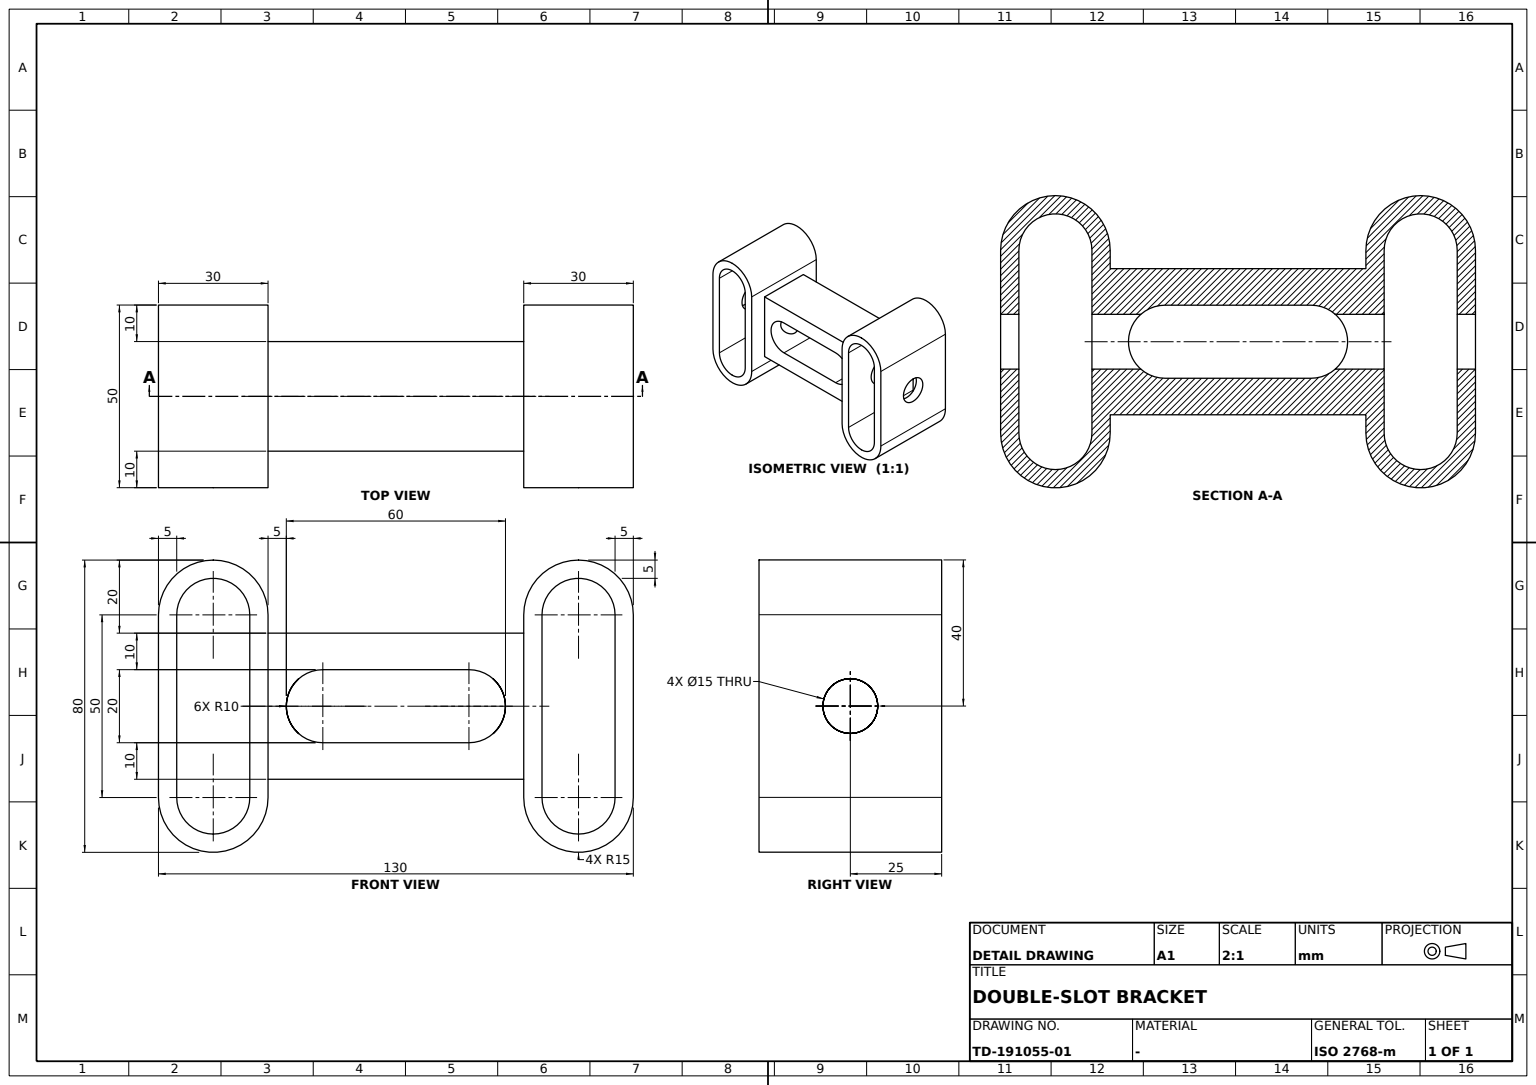
ISO-10303-21;
HEADER;
FILE_DESCRIPTION((''),'2;1');
FILE_NAME('','',(''),(''),'','','');
FILE_SCHEMA(('AUTOMOTIVE_DESIGN'));
ENDSEC;
DATA;
#1=APPLICATION_CONTEXT('');
#2=PRODUCT_CONTEXT('',#1,'mechanical');
#3=PRODUCT('','','',(#2));
#4=PRODUCT_DEFINITION_FORMATION('','',#3);
#5=PRODUCT_DEFINITION_CONTEXT('',#1,'design');
#6=PRODUCT_DEFINITION('','',#4,#5);
#7=PRODUCT_DEFINITION_SHAPE('','',#6);
#8=(LENGTH_UNIT()NAMED_UNIT(*)SI_UNIT(.MILLI.,.METRE.));
#9=(NAMED_UNIT(*)PLANE_ANGLE_UNIT()SI_UNIT($,.RADIAN.));
#10=(NAMED_UNIT(*)SI_UNIT($,.STERADIAN.)SOLID_ANGLE_UNIT());
#11=UNCERTAINTY_MEASURE_WITH_UNIT(LENGTH_MEASURE(0.005),#8,'distance_accuracy_value','');
#12=(GEOMETRIC_REPRESENTATION_CONTEXT(3)GLOBAL_UNCERTAINTY_ASSIGNED_CONTEXT((#11))GLOBAL_UNIT_ASSIGNED_CONTEXT((#8,#9,#10))REPRESENTATION_CONTEXT('',''));
#13=CARTESIAN_POINT('',(60.,-25.,25.));
#14=VERTEX_POINT('',#13);
#15=CARTESIAN_POINT('',(40.,-25.,25.));
#16=VERTEX_POINT('',#15);
#17=CARTESIAN_POINT('',(50.,-25.,25.));
#18=DIRECTION('',(0.,-1.,0.));
#19=DIRECTION('',(1.,0.,0.));
#20=AXIS2_PLACEMENT_3D('',#17,#18,#19);
#21=CIRCLE('',#20,10.);
#22=EDGE_CURVE('',#14,#16,#21,.T.);
#23=ORIENTED_EDGE('',*,*,#22,.F.);
#24=CARTESIAN_POINT('',(60.,-25.,-25.));
#25=VERTEX_POINT('',#24);
#26=DIRECTION('',(0.,0.,1.));
#27=VECTOR('',#26,1000.);
#28=LINE('',#24,#27);
#29=EDGE_CURVE('',#25,#14,#28,.T.);
#30=ORIENTED_EDGE('',*,*,#29,.F.);
#31=CARTESIAN_POINT('',(50.,-25.,-35.));
#32=VERTEX_POINT('',#31);
#33=CARTESIAN_POINT('',(50.,-25.,-25.));
#34=AXIS2_PLACEMENT_3D('',#33,#18,#19);
#35=CIRCLE('',#34,10.);
#36=EDGE_CURVE('',#32,#25,#35,.T.);
#37=ORIENTED_EDGE('',*,*,#36,.F.);
#38=CARTESIAN_POINT('',(40.,-25.,-25.));
#39=VERTEX_POINT('',#38);
#40=EDGE_CURVE('',#39,#32,#35,.T.);
#41=ORIENTED_EDGE('',*,*,#40,.F.);
#42=DIRECTION('',(0.,0.,-1.));
#43=VECTOR('',#42,1000.);
#44=LINE('',#15,#43);
#45=EDGE_CURVE('',#16,#39,#44,.T.);
#46=ORIENTED_EDGE('',*,*,#45,.F.);
#47=EDGE_LOOP('',(#23,#30,#37,#41,#46));
#48=FACE_BOUND('',#47,.T.);
#49=CARTESIAN_POINT('',(50.,-25.,40.));
#50=VERTEX_POINT('',#49);
#51=CARTESIAN_POINT('',(35.,-25.,25.));
#52=VERTEX_POINT('',#51);
#53=CIRCLE('',#20,15.);
#54=EDGE_CURVE('',#50,#52,#53,.T.);
#55=ORIENTED_EDGE('',*,*,#54,.T.);
#56=CARTESIAN_POINT('',(35.,-25.,-25.));
#57=VERTEX_POINT('',#56);
#58=LINE('',#51,#43);
#59=EDGE_CURVE('',#52,#57,#58,.T.);
#60=ORIENTED_EDGE('',*,*,#59,.T.);
#61=CARTESIAN_POINT('',(65.,-25.,-25.));
#62=VERTEX_POINT('',#61);
#63=CIRCLE('',#34,15.);
#64=EDGE_CURVE('',#57,#62,#63,.T.);
#65=ORIENTED_EDGE('',*,*,#64,.T.);
#66=CARTESIAN_POINT('',(65.,-25.,25.));
#67=VERTEX_POINT('',#66);
#68=LINE('',#61,#27);
#69=EDGE_CURVE('',#62,#67,#68,.T.);
#70=ORIENTED_EDGE('',*,*,#69,.T.);
#71=EDGE_CURVE('',#67,#50,#53,.T.);
#72=ORIENTED_EDGE('',*,*,#71,.T.);
#73=EDGE_LOOP('',(#55,#60,#65,#70,#72));
#74=FACE_BOUND('',#73,.T.);
#75=AXIS2_PLACEMENT_3D('',#33,#18,#42);
#76=PLANE('',#75);
#77=ADVANCED_FACE('',(#48,#74),#76,.T.);
#78=CARTESIAN_POINT('',(-60.,-25.,-25.));
#79=VERTEX_POINT('',#78);
#80=CARTESIAN_POINT('',(-60.,25.,-25.));
#81=VERTEX_POINT('',#80);
#82=DIRECTION('',(0.,1.,0.));
#83=VECTOR('',#82,1000.);
#84=LINE('',#80,#83);
#85=EDGE_CURVE('',#79,#81,#84,.T.);
#86=ORIENTED_EDGE('',*,*,#85,.T.);
#87=CARTESIAN_POINT('',(-60.,25.,25.));
#88=VERTEX_POINT('',#87);
#89=LINE('',#87,#43);
#90=EDGE_CURVE('',#88,#81,#89,.T.);
#91=ORIENTED_EDGE('',*,*,#90,.F.);
#92=CARTESIAN_POINT('',(-60.,-25.,25.));
#93=VERTEX_POINT('',#92);
#94=LINE('',#87,#83);
#95=EDGE_CURVE('',#93,#88,#94,.T.);
#96=ORIENTED_EDGE('',*,*,#95,.F.);
#97=LINE('',#92,#43);
#98=EDGE_CURVE('',#93,#79,#97,.T.);
#99=ORIENTED_EDGE('',*,*,#98,.T.);
#100=EDGE_LOOP('',(#86,#91,#96,#99));
#101=FACE_BOUND('',#100,.T.);
#102=CARTESIAN_POINT('',(-60.,0.,7.5));
#103=VERTEX_POINT('',#102);
#104=CARTESIAN_POINT('',(-60.,0.,-7.5));
#105=VERTEX_POINT('',#104);
#106=CARTESIAN_POINT('',(-60.,0.,0.));
#107=DIRECTION('',(-1.,0.,0.));
#108=AXIS2_PLACEMENT_3D('',#106,#107,#26);
#109=CIRCLE('',#108,7.5);
#110=EDGE_CURVE('',#103,#105,#109,.T.);
#111=ORIENTED_EDGE('',*,*,#110,.T.);
#112=EDGE_CURVE('',#105,#103,#109,.T.);
#113=ORIENTED_EDGE('',*,*,#112,.T.);
#114=EDGE_LOOP('',(#111,#113));
#115=FACE_BOUND('',#114,.T.);
#116=AXIS2_PLACEMENT_3D('',#87,#107,#26);
#117=PLANE('',#116);
#118=ADVANCED_FACE('',(#101,#115),#117,.F.);
#119=ORIENTED_EDGE('',*,*,#64,.F.);
#120=CARTESIAN_POINT('',(35.,25.,-25.));
#121=VERTEX_POINT('',#120);
#122=LINE('',#56,#83);
#123=EDGE_CURVE('',#57,#121,#122,.T.);
#124=ORIENTED_EDGE('',*,*,#123,.T.);
#125=CARTESIAN_POINT('',(65.,25.,-25.));
#126=VERTEX_POINT('',#125);
#127=CARTESIAN_POINT('',(50.,25.,-25.));
#128=AXIS2_PLACEMENT_3D('',#127,#18,#19);
#129=CIRCLE('',#128,15.);
#130=EDGE_CURVE('',#121,#126,#129,.T.);
#131=ORIENTED_EDGE('',*,*,#130,.T.);
#132=LINE('',#61,#83);
#133=EDGE_CURVE('',#62,#126,#132,.T.);
#134=ORIENTED_EDGE('',*,*,#133,.F.);
#135=EDGE_LOOP('',(#119,#124,#131,#134));
#136=FACE_BOUND('',#135,.T.);
#137=AXIS2_PLACEMENT_3D('',#33,#82,#26);
#138=CYLINDRICAL_SURFACE('',#137,15.);
#139=ADVANCED_FACE('',(#136),#138,.T.);
#140=CARTESIAN_POINT('',(-65.,0.,-7.5));
#141=VERTEX_POINT('',#140);
#142=CARTESIAN_POINT('',(-54935.,0.,-7.5));
#143=VECTOR('',#19,1000.);
#144=LINE('',#142,#143);
#145=EDGE_CURVE('',#141,#105,#144,.T.);
#146=ORIENTED_EDGE('',*,*,#145,.T.);
#147=ORIENTED_EDGE('',*,*,#110,.F.);
#148=CARTESIAN_POINT('',(-65.,0.,7.5));
#149=VERTEX_POINT('',#148);
#150=CARTESIAN_POINT('',(-54935.,0.,7.5));
#151=LINE('',#150,#143);
#152=EDGE_CURVE('',#103,#149,#151,.F.);
#153=ORIENTED_EDGE('',*,*,#152,.T.);
#154=CARTESIAN_POINT('',(-65.,0.,0.));
#155=AXIS2_PLACEMENT_3D('',#154,#19,#42);
#156=CIRCLE('',#155,7.5);
#157=EDGE_CURVE('',#141,#149,#156,.T.);
#158=ORIENTED_EDGE('',*,*,#157,.F.);
#159=EDGE_LOOP('',(#146,#147,#153,#158));
#160=FACE_BOUND('',#159,.T.);
#161=CARTESIAN_POINT('',(-54935.,0.,0.));
#162=AXIS2_PLACEMENT_3D('',#161,#19,#42);
#163=CYLINDRICAL_SURFACE('',#162,7.5);
#164=ADVANCED_FACE('',(#160),#163,.F.);
#165=CARTESIAN_POINT('',(-35.,-25.,-25.));
#166=VERTEX_POINT('',#165);
#167=CARTESIAN_POINT('',(-35.,25.,-25.));
#168=VERTEX_POINT('',#167);
#169=LINE('',#165,#83);
#170=EDGE_CURVE('',#166,#168,#169,.T.);
#171=ORIENTED_EDGE('',*,*,#170,.T.);
#172=CARTESIAN_POINT('',(-35.,25.,25.));
#173=VERTEX_POINT('',#172);
#174=LINE('',#167,#27);
#175=EDGE_CURVE('',#168,#173,#174,.T.);
#176=ORIENTED_EDGE('',*,*,#175,.T.);
#177=CARTESIAN_POINT('',(-35.,-25.,25.));
#178=VERTEX_POINT('',#177);
#179=LINE('',#177,#83);
#180=EDGE_CURVE('',#178,#173,#179,.T.);
#181=ORIENTED_EDGE('',*,*,#180,.F.);
#182=LINE('',#165,#27);
#183=EDGE_CURVE('',#166,#178,#182,.T.);
#184=ORIENTED_EDGE('',*,*,#183,.F.);
#185=EDGE_LOOP('',(#171,#176,#181,#184));
#186=FACE_BOUND('',#185,.T.);
#187=CARTESIAN_POINT('',(-35.,-15.,20.));
#188=VERTEX_POINT('',#187);
#189=CARTESIAN_POINT('',(-35.,-15.,-20.));
#190=VERTEX_POINT('',#189);
#191=LINE('',#187,#43);
#192=EDGE_CURVE('',#188,#190,#191,.T.);
#193=ORIENTED_EDGE('',*,*,#192,.F.);
#194=CARTESIAN_POINT('',(-35.,15.,20.));
#195=VERTEX_POINT('',#194);
#196=LINE('',#187,#83);
#197=EDGE_CURVE('',#188,#195,#196,.T.);
#198=ORIENTED_EDGE('',*,*,#197,.T.);
#199=CARTESIAN_POINT('',(-35.,15.,-20.));
#200=VERTEX_POINT('',#199);
#201=LINE('',#194,#43);
#202=EDGE_CURVE('',#195,#200,#201,.T.);
#203=ORIENTED_EDGE('',*,*,#202,.T.);
#204=LINE('',#189,#83);
#205=EDGE_CURVE('',#190,#200,#204,.T.);
#206=ORIENTED_EDGE('',*,*,#205,.F.);
#207=EDGE_LOOP('',(#193,#198,#203,#206));
#208=FACE_BOUND('',#207,.T.);
#209=AXIS2_PLACEMENT_3D('',#165,#107,#26);
#210=PLANE('',#209);
#211=ADVANCED_FACE('',(#186,#208),#210,.F.);
#212=CARTESIAN_POINT('',(60.,0.,-7.5));
#213=VERTEX_POINT('',#212);
#214=CARTESIAN_POINT('',(60.,0.,7.5));
#215=VERTEX_POINT('',#214);
#216=CARTESIAN_POINT('',(60.,0.,0.));
#217=AXIS2_PLACEMENT_3D('',#216,#19,#42);
#218=CIRCLE('',#217,7.5);
#219=EDGE_CURVE('',#213,#215,#218,.T.);
#220=ORIENTED_EDGE('',*,*,#219,.T.);
#221=EDGE_CURVE('',#215,#213,#218,.T.);
#222=ORIENTED_EDGE('',*,*,#221,.T.);
#223=EDGE_LOOP('',(#220,#222));
#224=FACE_BOUND('',#223,.T.);
#225=ORIENTED_EDGE('',*,*,#29,.T.);
#226=CARTESIAN_POINT('',(60.,25.,25.));
#227=VERTEX_POINT('',#226);
#228=LINE('',#226,#83);
#229=EDGE_CURVE('',#14,#227,#228,.T.);
#230=ORIENTED_EDGE('',*,*,#229,.T.);
#231=CARTESIAN_POINT('',(60.,25.,-25.));
#232=VERTEX_POINT('',#231);
#233=LINE('',#231,#27);
#234=EDGE_CURVE('',#232,#227,#233,.T.);
#235=ORIENTED_EDGE('',*,*,#234,.F.);
#236=LINE('',#231,#83);
#237=EDGE_CURVE('',#25,#232,#236,.T.);
#238=ORIENTED_EDGE('',*,*,#237,.F.);
#239=EDGE_LOOP('',(#225,#230,#235,#238));
#240=FACE_BOUND('',#239,.T.);
#241=AXIS2_PLACEMENT_3D('',#231,#19,#42);
#242=PLANE('',#241);
#243=ADVANCED_FACE('',(#224,#240),#242,.F.);
#244=CARTESIAN_POINT('',(65.,0.,7.5));
#245=VERTEX_POINT('',#244);
#246=CARTESIAN_POINT('',(65.,0.,-7.5));
#247=VERTEX_POINT('',#246);
#248=CARTESIAN_POINT('',(65.,0.,0.));
#249=AXIS2_PLACEMENT_3D('',#248,#19,#82);
#250=CIRCLE('',#249,7.5);
#251=EDGE_CURVE('',#245,#247,#250,.T.);
#252=ORIENTED_EDGE('',*,*,#251,.F.);
#253=EDGE_CURVE('',#247,#245,#250,.T.);
#254=ORIENTED_EDGE('',*,*,#253,.F.);
#255=EDGE_LOOP('',(#252,#254));
#256=FACE_BOUND('',#255,.T.);
#257=ORIENTED_EDGE('',*,*,#69,.F.);
#258=ORIENTED_EDGE('',*,*,#133,.T.);
#259=CARTESIAN_POINT('',(65.,25.,25.));
#260=VERTEX_POINT('',#259);
#261=LINE('',#125,#27);
#262=EDGE_CURVE('',#126,#260,#261,.T.);
#263=ORIENTED_EDGE('',*,*,#262,.T.);
#264=LINE('',#66,#83);
#265=EDGE_CURVE('',#67,#260,#264,.T.);
#266=ORIENTED_EDGE('',*,*,#265,.F.);
#267=EDGE_LOOP('',(#257,#258,#263,#266));
#268=FACE_BOUND('',#267,.T.);
#269=AXIS2_PLACEMENT_3D('',#61,#107,#26);
#270=PLANE('',#269);
#271=ADVANCED_FACE('',(#256,#268),#270,.F.);
#272=CARTESIAN_POINT('',(50.,25.,40.));
#273=VERTEX_POINT('',#272);
#274=LINE('',#49,#83);
#275=EDGE_CURVE('',#50,#273,#274,.T.);
#276=ORIENTED_EDGE('',*,*,#275,.F.);
#277=ORIENTED_EDGE('',*,*,#71,.F.);
#278=ORIENTED_EDGE('',*,*,#265,.T.);
#279=CARTESIAN_POINT('',(50.,25.,25.));
#280=AXIS2_PLACEMENT_3D('',#279,#18,#19);
#281=CIRCLE('',#280,15.);
#282=EDGE_CURVE('',#260,#273,#281,.T.);
#283=ORIENTED_EDGE('',*,*,#282,.T.);
#284=EDGE_LOOP('',(#276,#277,#278,#283));
#285=FACE_BOUND('',#284,.T.);
#286=AXIS2_PLACEMENT_3D('',#17,#82,#26);
#287=CYLINDRICAL_SURFACE('',#286,15.);
#288=ADVANCED_FACE('',(#285),#287,.T.);
#289=CARTESIAN_POINT('',(-50.,25.,40.));
#290=VERTEX_POINT('',#289);
#291=CARTESIAN_POINT('',(-65.,25.,25.));
#292=VERTEX_POINT('',#291);
#293=CARTESIAN_POINT('',(-50.,25.,25.));
#294=AXIS2_PLACEMENT_3D('',#293,#18,#19);
#295=CIRCLE('',#294,15.);
#296=EDGE_CURVE('',#290,#292,#295,.T.);
#297=ORIENTED_EDGE('',*,*,#296,.T.);
#298=CARTESIAN_POINT('',(-65.,-25.,25.));
#299=VERTEX_POINT('',#298);
#300=LINE('',#298,#83);
#301=EDGE_CURVE('',#299,#292,#300,.T.);
#302=ORIENTED_EDGE('',*,*,#301,.F.);
#303=CARTESIAN_POINT('',(-50.,-25.,40.));
#304=VERTEX_POINT('',#303);
#305=CARTESIAN_POINT('',(-50.,-25.,25.));
#306=AXIS2_PLACEMENT_3D('',#305,#18,#19);
#307=CIRCLE('',#306,15.);
#308=EDGE_CURVE('',#304,#299,#307,.T.);
#309=ORIENTED_EDGE('',*,*,#308,.F.);
#310=LINE('',#303,#83);
#311=EDGE_CURVE('',#304,#290,#310,.T.);
#312=ORIENTED_EDGE('',*,*,#311,.T.);
#313=EDGE_LOOP('',(#297,#302,#309,#312));
#314=FACE_BOUND('',#313,.T.);
#315=AXIS2_PLACEMENT_3D('',#305,#82,#26);
#316=CYLINDRICAL_SURFACE('',#315,15.);
#317=ADVANCED_FACE('',(#314),#316,.T.);
#318=CARTESIAN_POINT('',(20.,15.,10.));
#319=VERTEX_POINT('',#318);
#320=CARTESIAN_POINT('',(-20.,15.,10.));
#321=VERTEX_POINT('',#320);
#322=VECTOR('',#107,1000.);
#323=LINE('',#318,#322);
#324=EDGE_CURVE('',#319,#321,#323,.T.);
#325=ORIENTED_EDGE('',*,*,#324,.F.);
#326=CARTESIAN_POINT('',(20.,-15.,10.));
#327=VERTEX_POINT('',#326);
#328=LINE('',#318,#83);
#329=EDGE_CURVE('',#327,#319,#328,.T.);
#330=ORIENTED_EDGE('',*,*,#329,.F.);
#331=CARTESIAN_POINT('',(-20.,-15.,10.));
#332=VERTEX_POINT('',#331);
#333=LINE('',#326,#322);
#334=EDGE_CURVE('',#327,#332,#333,.T.);
#335=ORIENTED_EDGE('',*,*,#334,.T.);
#336=LINE('',#320,#83);
#337=EDGE_CURVE('',#332,#321,#336,.T.);
#338=ORIENTED_EDGE('',*,*,#337,.T.);
#339=EDGE_LOOP('',(#325,#330,#335,#338));
#340=FACE_BOUND('',#339,.T.);
#341=AXIS2_PLACEMENT_3D('',#318,#26,#19);
#342=PLANE('',#341);
#343=ADVANCED_FACE('',(#340),#342,.F.);
#344=CARTESIAN_POINT('',(35.,25.,25.));
#345=VERTEX_POINT('',#344);
#346=LINE('',#51,#83);
#347=EDGE_CURVE('',#52,#345,#346,.T.);
#348=ORIENTED_EDGE('',*,*,#347,.T.);
#349=LINE('',#344,#43);
#350=EDGE_CURVE('',#345,#121,#349,.T.);
#351=ORIENTED_EDGE('',*,*,#350,.T.);
#352=ORIENTED_EDGE('',*,*,#123,.F.);
#353=ORIENTED_EDGE('',*,*,#59,.F.);
#354=EDGE_LOOP('',(#348,#351,#352,#353));
#355=FACE_BOUND('',#354,.T.);
#356=CARTESIAN_POINT('',(35.,-15.,20.));
#357=VERTEX_POINT('',#356);
#358=CARTESIAN_POINT('',(35.,15.,20.));
#359=VERTEX_POINT('',#358);
#360=LINE('',#356,#83);
#361=EDGE_CURVE('',#357,#359,#360,.T.);
#362=ORIENTED_EDGE('',*,*,#361,.F.);
#363=CARTESIAN_POINT('',(35.,-15.,-20.));
#364=VERTEX_POINT('',#363);
#365=LINE('',#363,#27);
#366=EDGE_CURVE('',#364,#357,#365,.T.);
#367=ORIENTED_EDGE('',*,*,#366,.F.);
#368=CARTESIAN_POINT('',(35.,15.,-20.));
#369=VERTEX_POINT('',#368);
#370=LINE('',#363,#83);
#371=EDGE_CURVE('',#364,#369,#370,.T.);
#372=ORIENTED_EDGE('',*,*,#371,.T.);
#373=LINE('',#368,#27);
#374=EDGE_CURVE('',#369,#359,#373,.T.);
#375=ORIENTED_EDGE('',*,*,#374,.T.);
#376=EDGE_LOOP('',(#362,#367,#372,#375));
#377=FACE_BOUND('',#376,.T.);
#378=AXIS2_PLACEMENT_3D('',#51,#19,#42);
#379=PLANE('',#378);
#380=ADVANCED_FACE('',(#355,#377),#379,.F.);
#381=CARTESIAN_POINT('',(-65.,-25.,-25.));
#382=VERTEX_POINT('',#381);
#383=CARTESIAN_POINT('',(-65.,25.,-25.));
#384=VERTEX_POINT('',#383);
#385=LINE('',#381,#83);
#386=EDGE_CURVE('',#382,#384,#385,.T.);
#387=ORIENTED_EDGE('',*,*,#386,.T.);
#388=CARTESIAN_POINT('',(-50.,25.,-25.));
#389=AXIS2_PLACEMENT_3D('',#388,#18,#19);
#390=CIRCLE('',#389,15.);
#391=EDGE_CURVE('',#384,#168,#390,.T.);
#392=ORIENTED_EDGE('',*,*,#391,.T.);
#393=ORIENTED_EDGE('',*,*,#170,.F.);
#394=CARTESIAN_POINT('',(-50.,-25.,-25.));
#395=AXIS2_PLACEMENT_3D('',#394,#18,#19);
#396=CIRCLE('',#395,15.);
#397=EDGE_CURVE('',#382,#166,#396,.T.);
#398=ORIENTED_EDGE('',*,*,#397,.F.);
#399=EDGE_LOOP('',(#387,#392,#393,#398));
#400=FACE_BOUND('',#399,.T.);
#401=AXIS2_PLACEMENT_3D('',#394,#82,#26);
#402=CYLINDRICAL_SURFACE('',#401,15.);
#403=ADVANCED_FACE('',(#400),#402,.T.);
#404=CARTESIAN_POINT('',(-40.,0.,-7.5));
#405=VERTEX_POINT('',#404);
#406=CARTESIAN_POINT('',(-40.,0.,7.5));
#407=VERTEX_POINT('',#406);
#408=CARTESIAN_POINT('',(-40.,0.,0.));
#409=AXIS2_PLACEMENT_3D('',#408,#19,#42);
#410=CIRCLE('',#409,7.5);
#411=EDGE_CURVE('',#405,#407,#410,.T.);
#412=ORIENTED_EDGE('',*,*,#411,.T.);
#413=EDGE_CURVE('',#407,#405,#410,.T.);
#414=ORIENTED_EDGE('',*,*,#413,.T.);
#415=EDGE_LOOP('',(#412,#414));
#416=FACE_BOUND('',#415,.T.);
#417=CARTESIAN_POINT('',(-40.,-25.,-25.));
#418=VERTEX_POINT('',#417);
#419=CARTESIAN_POINT('',(-40.,25.,-25.));
#420=VERTEX_POINT('',#419);
#421=LINE('',#419,#83);
#422=EDGE_CURVE('',#418,#420,#421,.T.);
#423=ORIENTED_EDGE('',*,*,#422,.F.);
#424=CARTESIAN_POINT('',(-40.,-25.,25.));
#425=VERTEX_POINT('',#424);
#426=LINE('',#417,#27);
#427=EDGE_CURVE('',#418,#425,#426,.T.);
#428=ORIENTED_EDGE('',*,*,#427,.T.);
#429=CARTESIAN_POINT('',(-40.,25.,25.));
#430=VERTEX_POINT('',#429);
#431=LINE('',#429,#83);
#432=EDGE_CURVE('',#425,#430,#431,.T.);
#433=ORIENTED_EDGE('',*,*,#432,.T.);
#434=LINE('',#419,#27);
#435=EDGE_CURVE('',#420,#430,#434,.T.);
#436=ORIENTED_EDGE('',*,*,#435,.F.);
#437=EDGE_LOOP('',(#423,#428,#433,#436));
#438=FACE_BOUND('',#437,.T.);
#439=AXIS2_PLACEMENT_3D('',#419,#19,#42);
#440=PLANE('',#439);
#441=ADVANCED_FACE('',(#416,#438),#440,.F.);
#442=LINE('',#298,#43);
#443=EDGE_CURVE('',#299,#382,#442,.T.);
#444=ORIENTED_EDGE('',*,*,#443,.T.);
#445=ORIENTED_EDGE('',*,*,#397,.T.);
#446=ORIENTED_EDGE('',*,*,#183,.T.);
#447=EDGE_CURVE('',#178,#304,#307,.T.);
#448=ORIENTED_EDGE('',*,*,#447,.T.);
#449=ORIENTED_EDGE('',*,*,#308,.T.);
#450=EDGE_LOOP('',(#444,#445,#446,#448,#449));
#451=FACE_BOUND('',#450,.T.);
#452=CARTESIAN_POINT('',(-50.,-25.,-35.));
#453=VERTEX_POINT('',#452);
#454=CIRCLE('',#395,10.);
#455=EDGE_CURVE('',#79,#453,#454,.T.);
#456=ORIENTED_EDGE('',*,*,#455,.F.);
#457=ORIENTED_EDGE('',*,*,#98,.F.);
#458=CIRCLE('',#306,10.);
#459=EDGE_CURVE('',#425,#93,#458,.T.);
#460=ORIENTED_EDGE('',*,*,#459,.F.);
#461=ORIENTED_EDGE('',*,*,#427,.F.);
#462=EDGE_CURVE('',#453,#418,#454,.T.);
#463=ORIENTED_EDGE('',*,*,#462,.F.);
#464=EDGE_LOOP('',(#456,#457,#460,#461,#463));
#465=FACE_BOUND('',#464,.T.);
#466=AXIS2_PLACEMENT_3D('',#394,#18,#42);
#467=PLANE('',#466);
#468=ADVANCED_FACE('',(#451,#465),#467,.T.);
#469=ORIENTED_EDGE('',*,*,#202,.F.);
#470=LINE('',#358,#322);
#471=EDGE_CURVE('',#359,#195,#470,.T.);
#472=ORIENTED_EDGE('',*,*,#471,.F.);
#473=ORIENTED_EDGE('',*,*,#374,.F.);
#474=LINE('',#199,#143);
#475=EDGE_CURVE('',#200,#369,#474,.T.);
#476=ORIENTED_EDGE('',*,*,#475,.F.);
#477=EDGE_LOOP('',(#469,#472,#473,#476));
#478=FACE_BOUND('',#477,.T.);
#479=ORIENTED_EDGE('',*,*,#324,.T.);
#480=CARTESIAN_POINT('',(-20.,15.,-10.));
#481=VERTEX_POINT('',#480);
#482=CARTESIAN_POINT('',(-20.,15.,0.));
#483=AXIS2_PLACEMENT_3D('',#482,#18,#19);
#484=CIRCLE('',#483,10.);
#485=EDGE_CURVE('',#321,#481,#484,.T.);
#486=ORIENTED_EDGE('',*,*,#485,.T.);
#487=CARTESIAN_POINT('',(20.,15.,-10.));
#488=VERTEX_POINT('',#487);
#489=LINE('',#480,#143);
#490=EDGE_CURVE('',#481,#488,#489,.T.);
#491=ORIENTED_EDGE('',*,*,#490,.T.);
#492=CARTESIAN_POINT('',(20.,15.,0.));
#493=AXIS2_PLACEMENT_3D('',#492,#18,#19);
#494=CIRCLE('',#493,10.);
#495=EDGE_CURVE('',#488,#319,#494,.T.);
#496=ORIENTED_EDGE('',*,*,#495,.T.);
#497=EDGE_LOOP('',(#479,#486,#491,#496));
#498=FACE_BOUND('',#497,.T.);
#499=CARTESIAN_POINT('',(0.,15.,0.));
#500=AXIS2_PLACEMENT_3D('',#499,#18,#42);
#501=PLANE('',#500);
#502=ADVANCED_FACE('',(#478,#498),#501,.F.);
#503=ORIENTED_EDGE('',*,*,#54,.F.);
#504=ORIENTED_EDGE('',*,*,#275,.T.);
#505=EDGE_CURVE('',#273,#345,#281,.T.);
#506=ORIENTED_EDGE('',*,*,#505,.T.);
#507=ORIENTED_EDGE('',*,*,#347,.F.);
#508=EDGE_LOOP('',(#503,#504,#506,#507));
#509=FACE_BOUND('',#508,.T.);
#510=ADVANCED_FACE('',(#509),#287,.T.);
#511=CARTESIAN_POINT('',(-26.614378,0.,7.5));
#512=VERTEX_POINT('',#511);
#513=CARTESIAN_POINT('',(-26.614378,0.,-7.5));
#514=VERTEX_POINT('',#513);
#515=CARTESIAN_POINT('',(-26.614378,0.249532,-7.5));
#516=CARTESIAN_POINT('',(-26.641461,0.748413,-7.476904));
#517=CARTESIAN_POINT('',(-26.757864,1.419399,-7.371557));
#518=CARTESIAN_POINT('',(-26.873798,1.88168,-7.263436));
#519=CARTESIAN_POINT('',(-26.988253,2.263769,-7.153239));
#520=CARTESIAN_POINT('',(-27.09675,2.578479,-7.046079));
#521=CARTESIAN_POINT('',(-27.240211,2.949846,-6.898634));
#522=CARTESIAN_POINT('',(-27.364001,3.241305,-6.766688));
#523=CARTESIAN_POINT('',(-27.529484,3.601545,-6.582138));
#524=CARTESIAN_POINT('',(-27.638212,3.821161,-6.454985));
#525=CARTESIAN_POINT('',(-27.74168,4.023868,-6.330447));
#526=CARTESIAN_POINT('',(-27.839375,4.208389,-6.208747));
#527=CARTESIAN_POINT('',(-27.883153,4.288939,-6.15293));
#528=CARTESIAN_POINT('',(-27.982001,4.469189,-6.02534));
#529=CARTESIAN_POINT('',(-28.146542,4.758555,-5.802902));
#530=CARTESIAN_POINT('',(-28.306341,5.025628,-5.569646));
#531=CARTESIAN_POINT('',(-28.406734,5.188969,-5.415587));
#532=CARTESIAN_POINT('',(-28.452686,5.263124,-5.344101));
#533=CARTESIAN_POINT('',(-28.553383,5.423668,-5.181742));
#534=CARTESIAN_POINT('',(-28.662057,5.593914,-4.998258));
#535=CARTESIAN_POINT('',(-28.794253,5.797092,-4.763522));
#536=CARTESIAN_POINT('',(-28.938334,6.012716,-4.486266));
#537=CARTESIAN_POINT('',(-29.052554,6.180973,-4.252798));
#538=CARTESIAN_POINT('',(-29.206854,6.405149,-3.909033));
#539=CARTESIAN_POINT('',(-29.378054,6.649219,-3.482672));
#540=CARTESIAN_POINT('',(-29.557088,6.899236,-2.973028));
#541=CARTESIAN_POINT('',(-29.759051,7.176399,-2.223888));
#542=CARTESIAN_POINT('',(-29.892448,7.356079,-1.523956));
#543=CARTESIAN_POINT('',(-29.982333,7.476665,-0.745859));
#544=CARTESIAN_POINT('',(-30.009395,7.512415,0.01454));
#545=CARTESIAN_POINT('',(-29.980018,7.473584,0.77805));
#546=CARTESIAN_POINT('',(-29.886857,7.348565,1.559605));
#547=CARTESIAN_POINT('',(-29.751815,7.166582,2.255496));
#548=CARTESIAN_POINT('',(-29.54649,6.88456,3.00652));
#549=CARTESIAN_POINT('',(-29.369647,6.637331,3.504846));
#550=CARTESIAN_POINT('',(-29.199801,6.394989,3.925434));
#551=CARTESIAN_POINT('',(-29.047679,6.173824,4.263065));
#552=CARTESIAN_POINT('',(-28.933161,6.005025,4.496569));
#553=CARTESIAN_POINT('',(-28.789456,5.78981,4.772334));
#554=CARTESIAN_POINT('',(-28.657359,5.586636,5.006375));
#555=CARTESIAN_POINT('',(-28.54892,5.41663,5.189099));
#556=CARTESIAN_POINT('',(-28.448049,5.25567,5.351424));
#557=CARTESIAN_POINT('',(-28.403238,5.183297,5.420994));
#558=CARTESIAN_POINT('',(-28.3034,5.020789,5.574017));
#559=CARTESIAN_POINT('',(-28.142619,4.751854,5.808377));
#560=CARTESIAN_POINT('',(-27.979385,4.46453,6.02878));
#561=CARTESIAN_POINT('',(-27.880063,4.283274,6.156893));
#562=CARTESIAN_POINT('',(-27.835163,4.200543,6.214066));
#563=CARTESIAN_POINT('',(-27.737542,4.015903,6.335502));
#564=CARTESIAN_POINT('',(-27.633823,3.812403,6.460185));
#565=CARTESIAN_POINT('',(-27.52428,3.590686,6.588076));
#566=CARTESIAN_POINT('',(-27.360602,3.233337,6.770341));
#567=CARTESIAN_POINT('',(-27.239782,2.948976,6.899043));
#568=CARTESIAN_POINT('',(-27.089678,2.559863,7.053569));
#569=CARTESIAN_POINT('',(-26.971483,2.209834,7.170169));
#570=CARTESIAN_POINT('',(-26.867155,1.854135,7.269814));
#571=CARTESIAN_POINT('',(-26.787674,1.537805,7.343705));
#572=CARTESIAN_POINT('',(-26.707159,1.13393,7.417519));
#573=CARTESIAN_POINT('',(-26.636615,0.629284,7.480873));
#574=CARTESIAN_POINT('',(-26.614378,0.248681,7.5));
#575=B_SPLINE_CURVE_WITH_KNOTS('',3,(#513,#515,#516,#517,#518,#519,#520,#521,#522,#523,#524,#525,#526,#527,#528,#529,#530,#531,#532,#533,#534,#535,#536,#537,#538,#539,#540,#541,#542,#543,#544,#545,#546,#547,#548,#549,#550,#551,#552,#553,#554,#555,#556,#557,#558,#559,#560,#561,#562,#563,#564,#565,#566,#567,#568,#569,#570,#571,#572,#573,#574,#511),.UNSPECIFIED.,.F.,.F.,(4,1,1,1,1,1,1,1,1,1,1,1,1,1,1,1,1,1,1,1,1,1,1,1,1,1,1,1,1,1,1,1,1,1,1,1,1,1,1,1,1,1,1,1,1,1,1,1,1,1,1,1,1,1,1,1,1,1,1,4),(0.,0.03125,0.0625,0.078125,0.09375,0.109375,0.125,0.140625,0.15625,0.171875,0.1796875,0.1875,0.1953125,0.203125,0.21875,0.234375,0.2421875,0.25,0.2578125,0.265625,0.28125,0.296875,0.3125,0.328125,0.34375,0.375,0.40625,0.4375,0.46875,0.5,0.53125,0.5625,0.59375,0.625,0.65625,0.671875,0.6875,0.703125,0.71875,0.734375,0.7421875,0.75,0.7578125,0.765625,0.78125,0.796875,0.8046875,0.8125,0.8203125,0.828125,0.84375,0.859375,0.875,0.890625,0.90625,0.921875,0.9375,0.953125,0.96875,1.),.UNSPECIFIED.);
#576=EDGE_CURVE('',#512,#514,#575,.F.);
#577=ORIENTED_EDGE('',*,*,#576,.T.);
#578=CARTESIAN_POINT('',(-26.614399,-0.252132,-7.499982));
#579=CARTESIAN_POINT('',(-26.641932,-0.752085,-7.475958));
#580=CARTESIAN_POINT('',(-26.777233,-1.532111,-7.354135));
#581=CARTESIAN_POINT('',(-26.963933,-2.213142,-7.179093));
#582=CARTESIAN_POINT('',(-27.232077,-2.946301,-6.909931));
#583=CARTESIAN_POINT('',(-27.503526,-3.557066,-6.615558));
#584=CARTESIAN_POINT('',(-27.827407,-4.195732,-6.23051));
#585=CARTESIAN_POINT('',(-28.136234,-4.744765,-5.822204));
#586=CARTESIAN_POINT('',(-28.565389,-5.453737,-5.187209));
#587=CARTESIAN_POINT('',(-29.070321,-6.215527,-4.276677));
#588=CARTESIAN_POINT('',(-29.570523,-6.920886,-3.014154));
#589=CARTESIAN_POINT('',(-29.916491,-7.389274,-1.562867));
#590=CARTESIAN_POINT('',(-30.083236,-7.609974,0.502085));
#591=CARTESIAN_POINT('',(-29.668239,-7.063625,3.063079));
#592=CARTESIAN_POINT('',(-28.784203,-5.814048,4.861835));
#593=CARTESIAN_POINT('',(-28.141198,-4.753296,5.815307));
#594=CARTESIAN_POINT('',(-27.831958,-4.204194,6.22482));
#595=CARTESIAN_POINT('',(-27.507488,-3.565427,6.611097));
#596=CARTESIAN_POINT('',(-27.235149,-2.953864,6.906736));
#597=CARTESIAN_POINT('',(-26.966611,-2.221264,7.1765));
#598=CARTESIAN_POINT('',(-26.779465,-1.542274,7.352097));
#599=CARTESIAN_POINT('',(-26.642153,-0.756112,7.475775));
#600=CARTESIAN_POINT('',(-26.614399,-0.253607,7.499982));
#601=B_SPLINE_CURVE_WITH_KNOTS('',3,(#513,#578,#579,#580,#581,#582,#583,#584,#585,#586,#587,#588,#589,#590,#591,#592,#593,#594,#595,#596,#597,#598,#599,#600,#511),.UNSPECIFIED.,.F.,.F.,(4,1,1,1,1,1,1,1,1,1,1,1,1,1,1,1,1,1,1,1,1,1,4),(0.,0.03125,0.0625,0.09375,0.125,0.15625,0.1875,0.21875,0.25,0.3125,0.375,0.4375,0.5,0.625,0.75,0.78125,0.8125,0.84375,0.875,0.90625,0.9375,0.96875,1.),.UNSPECIFIED.);
#602=EDGE_CURVE('',#514,#512,#601,.T.);
#603=ORIENTED_EDGE('',*,*,#602,.T.);
#604=EDGE_LOOP('',(#577,#603));
#605=FACE_BOUND('',#604,.T.);
#606=ORIENTED_EDGE('',*,*,#337,.F.);
#607=CARTESIAN_POINT('',(-20.,-15.,-10.));
#608=VERTEX_POINT('',#607);
#609=CARTESIAN_POINT('',(-20.,-15.,0.));
#610=AXIS2_PLACEMENT_3D('',#609,#18,#19);
#611=CIRCLE('',#610,10.);
#612=EDGE_CURVE('',#332,#608,#611,.T.);
#613=ORIENTED_EDGE('',*,*,#612,.T.);
#614=LINE('',#480,#83);
#615=EDGE_CURVE('',#608,#481,#614,.T.);
#616=ORIENTED_EDGE('',*,*,#615,.T.);
#617=ORIENTED_EDGE('',*,*,#485,.F.);
#618=EDGE_LOOP('',(#606,#613,#616,#617));
#619=FACE_BOUND('',#618,.T.);
#620=AXIS2_PLACEMENT_3D('',#482,#18,#42);
#621=CYLINDRICAL_SURFACE('',#620,10.);
#622=ADVANCED_FACE('',(#605,#619),#621,.F.);
#623=CARTESIAN_POINT('',(26.614378,0.,7.5));
#624=VERTEX_POINT('',#623);
#625=CARTESIAN_POINT('',(40.,0.,7.5));
#626=VERTEX_POINT('',#625);
#627=EDGE_CURVE('',#624,#626,#151,.T.);
#628=ORIENTED_EDGE('',*,*,#627,.F.);
#629=CARTESIAN_POINT('',(26.614378,0.,-7.5));
#630=VERTEX_POINT('',#629);
#631=CARTESIAN_POINT('',(26.614378,0.248853,7.5));
#632=CARTESIAN_POINT('',(26.641383,0.746622,7.476962));
#633=CARTESIAN_POINT('',(26.756857,1.414582,7.372471));
#634=CARTESIAN_POINT('',(26.872694,1.877665,7.264492));
#635=CARTESIAN_POINT('',(26.987199,2.260446,7.154299));
#636=CARTESIAN_POINT('',(27.095719,2.575623,7.047124));
#637=CARTESIAN_POINT('',(27.239034,2.946961,6.899872));
#638=CARTESIAN_POINT('',(27.362839,3.238683,6.76793));
#639=CARTESIAN_POINT('',(27.527642,3.597775,6.584179));
#640=CARTESIAN_POINT('',(27.636337,3.817468,6.457176));
#641=CARTESIAN_POINT('',(27.740148,4.020939,6.332323));
#642=CARTESIAN_POINT('',(27.838503,4.206769,6.209854));
#643=CARTESIAN_POINT('',(27.88236,4.287483,6.153945));
#644=CARTESIAN_POINT('',(27.981389,4.4681,6.026149));
#645=CARTESIAN_POINT('',(28.145643,4.757019,5.804158));
#646=CARTESIAN_POINT('',(28.305705,5.024584,5.570593));
#647=CARTESIAN_POINT('',(28.40602,5.18781,5.416692));
#648=CARTESIAN_POINT('',(28.451714,5.261562,5.345639));
#649=CARTESIAN_POINT('',(28.552599,5.422433,5.183038));
#650=CARTESIAN_POINT('',(28.661354,5.592828,4.999474));
#651=CARTESIAN_POINT('',(28.793687,5.796237,4.764572));
#652=CARTESIAN_POINT('',(28.937876,6.012037,4.487179));
#653=CARTESIAN_POINT('',(29.052172,6.180413,4.253616));
#654=CARTESIAN_POINT('',(29.206541,6.4047,3.909772));
#655=CARTESIAN_POINT('',(29.377821,6.648892,3.483306));
#656=CARTESIAN_POINT('',(29.556948,6.899043,2.973491));
#657=CARTESIAN_POINT('',(29.758928,7.176233,2.224393));
#658=CARTESIAN_POINT('',(29.892346,7.355942,1.524664));
#659=CARTESIAN_POINT('',(29.982349,7.476687,0.745887));
#660=CARTESIAN_POINT('',(30.009404,7.512426,-0.014994));
#661=CARTESIAN_POINT('',(29.979964,7.473513,-0.778904));
#662=CARTESIAN_POINT('',(29.886651,7.348289,-1.560969));
#663=CARTESIAN_POINT('',(29.751469,7.166113,-2.256991));
#664=CARTESIAN_POINT('',(29.545998,6.883881,-3.008117));
#665=CARTESIAN_POINT('',(29.368869,6.636237,-3.506939));
#666=CARTESIAN_POINT('',(29.198796,6.393547,-3.927801));
#667=CARTESIAN_POINT('',(29.046371,6.171908,-4.265843));
#668=CARTESIAN_POINT('',(28.93193,6.003194,-4.499005));
#669=CARTESIAN_POINT('',(28.788179,5.787874,-4.774685));
#670=CARTESIAN_POINT('',(28.656038,5.58459,-5.008656));
#671=CARTESIAN_POINT('',(28.547577,5.41451,-5.191312));
#672=CARTESIAN_POINT('',(28.446609,5.253356,-5.353696));
#673=CARTESIAN_POINT('',(28.401982,5.18126,-5.422936));
#674=CARTESIAN_POINT('',(28.302164,5.018751,-5.575864));
#675=CARTESIAN_POINT('',(28.140771,4.748684,-5.81097));
#676=CARTESIAN_POINT('',(27.97812,4.462265,-6.030447));
#677=CARTESIAN_POINT('',(27.878745,4.280851,-6.158582));
#678=CARTESIAN_POINT('',(27.833649,4.197719,-6.215974));
#679=CARTESIAN_POINT('',(27.73605,4.01303,-6.337323));
#680=CARTESIAN_POINT('',(27.632262,3.809279,-6.462028));
#681=CARTESIAN_POINT('',(27.522763,3.587525,-6.589812));
#682=CARTESIAN_POINT('',(27.358583,3.228784,-6.772544));
#683=CARTESIAN_POINT('',(27.237422,2.9432,-6.901517));
#684=CARTESIAN_POINT('',(27.087493,2.553831,-7.055762));
#685=CARTESIAN_POINT('',(26.969378,2.203191,-7.172215));
#686=CARTESIAN_POINT('',(26.865275,1.847247,-7.271589));
#687=CARTESIAN_POINT('',(26.785808,1.529484,-7.345426));
#688=CARTESIAN_POINT('',(26.70629,1.128486,-7.418297));
#689=CARTESIAN_POINT('',(26.636371,0.626119,-7.48108));
#690=CARTESIAN_POINT('',(26.614378,0.247492,-7.5));
#691=B_SPLINE_CURVE_WITH_KNOTS('',3,(#623,#631,#632,#633,#634,#635,#636,#637,#638,#639,#640,#641,#642,#643,#644,#645,#646,#647,#648,#649,#650,#651,#652,#653,#654,#655,#656,#657,#658,#659,#660,#661,#662,#663,#664,#665,#666,#667,#668,#669,#670,#671,#672,#673,#674,#675,#676,#677,#678,#679,#680,#681,#682,#683,#684,#685,#686,#687,#688,#689,#690,#629),.UNSPECIFIED.,.F.,.F.,(4,1,1,1,1,1,1,1,1,1,1,1,1,1,1,1,1,1,1,1,1,1,1,1,1,1,1,1,1,1,1,1,1,1,1,1,1,1,1,1,1,1,1,1,1,1,1,1,1,1,1,1,1,1,1,1,1,1,1,4),(0.,0.03125,0.0625,0.078125,0.09375,0.109375,0.125,0.140625,0.15625,0.171875,0.1796875,0.1875,0.1953125,0.203125,0.21875,0.234375,0.2421875,0.25,0.2578125,0.265625,0.28125,0.296875,0.3125,0.328125,0.34375,0.375,0.40625,0.4375,0.46875,0.5,0.53125,0.5625,0.59375,0.625,0.65625,0.671875,0.6875,0.703125,0.71875,0.734375,0.7421875,0.75,0.7578125,0.765625,0.78125,0.796875,0.8046875,0.8125,0.8203125,0.828125,0.84375,0.859375,0.875,0.890625,0.90625,0.921875,0.9375,0.953125,0.96875,1.),.UNSPECIFIED.);
#692=EDGE_CURVE('',#630,#624,#691,.F.);
#693=ORIENTED_EDGE('',*,*,#692,.F.);
#694=CARTESIAN_POINT('',(40.,0.,-7.5));
#695=VERTEX_POINT('',#694);
#696=EDGE_CURVE('',#695,#630,#144,.F.);
#697=ORIENTED_EDGE('',*,*,#696,.F.);
#698=CARTESIAN_POINT('',(40.,0.,0.));
#699=AXIS2_PLACEMENT_3D('',#698,#107,#26);
#700=CIRCLE('',#699,7.5);
#701=EDGE_CURVE('',#626,#695,#700,.T.);
#702=ORIENTED_EDGE('',*,*,#701,.F.);
#703=EDGE_LOOP('',(#628,#693,#697,#702));
#704=FACE_BOUND('',#703,.T.);
#705=ADVANCED_FACE('',(#704),#163,.F.);
#706=LINE('',#189,#143);
#707=EDGE_CURVE('',#190,#364,#706,.T.);
#708=ORIENTED_EDGE('',*,*,#707,.T.);
#709=ORIENTED_EDGE('',*,*,#366,.T.);
#710=LINE('',#356,#322);
#711=EDGE_CURVE('',#357,#188,#710,.T.);
#712=ORIENTED_EDGE('',*,*,#711,.T.);
#713=ORIENTED_EDGE('',*,*,#192,.T.);
#714=EDGE_LOOP('',(#708,#709,#712,#713));
#715=FACE_BOUND('',#714,.T.);
#716=ORIENTED_EDGE('',*,*,#334,.F.);
#717=CARTESIAN_POINT('',(20.,-15.,-10.));
#718=VERTEX_POINT('',#717);
#719=CARTESIAN_POINT('',(20.,-15.,0.));
#720=AXIS2_PLACEMENT_3D('',#719,#18,#19);
#721=CIRCLE('',#720,10.);
#722=EDGE_CURVE('',#718,#327,#721,.T.);
#723=ORIENTED_EDGE('',*,*,#722,.F.);
#724=LINE('',#607,#143);
#725=EDGE_CURVE('',#608,#718,#724,.T.);
#726=ORIENTED_EDGE('',*,*,#725,.F.);
#727=ORIENTED_EDGE('',*,*,#612,.F.);
#728=EDGE_LOOP('',(#716,#723,#726,#727));
#729=FACE_BOUND('',#728,.T.);
#730=CARTESIAN_POINT('',(0.,-15.,0.));
#731=AXIS2_PLACEMENT_3D('',#730,#18,#42);
#732=PLANE('',#731);
#733=ADVANCED_FACE('',(#715,#729),#732,.T.);
#734=ORIENTED_EDGE('',*,*,#40,.T.);
#735=CARTESIAN_POINT('',(50.,25.,-35.));
#736=VERTEX_POINT('',#735);
#737=VECTOR('',#18,1000.);
#738=LINE('',#735,#737);
#739=EDGE_CURVE('',#736,#32,#738,.T.);
#740=ORIENTED_EDGE('',*,*,#739,.F.);
#741=CARTESIAN_POINT('',(40.,25.,-25.));
#742=VERTEX_POINT('',#741);
#743=CIRCLE('',#128,10.);
#744=EDGE_CURVE('',#742,#736,#743,.T.);
#745=ORIENTED_EDGE('',*,*,#744,.F.);
#746=LINE('',#741,#83);
#747=EDGE_CURVE('',#39,#742,#746,.T.);
#748=ORIENTED_EDGE('',*,*,#747,.F.);
#749=EDGE_LOOP('',(#734,#740,#745,#748));
#750=FACE_BOUND('',#749,.T.);
#751=AXIS2_PLACEMENT_3D('',#127,#18,#42);
#752=CYLINDRICAL_SURFACE('',#751,10.);
#753=ADVANCED_FACE('',(#750),#752,.F.);
#754=ORIENTED_EDGE('',*,*,#180,.T.);
#755=EDGE_CURVE('',#173,#290,#295,.T.);
#756=ORIENTED_EDGE('',*,*,#755,.T.);
#757=ORIENTED_EDGE('',*,*,#311,.F.);
#758=ORIENTED_EDGE('',*,*,#447,.F.);
#759=EDGE_LOOP('',(#754,#756,#757,#758));
#760=FACE_BOUND('',#759,.T.);
#761=ADVANCED_FACE('',(#760),#316,.T.);
#762=CARTESIAN_POINT('',(40.,25.,25.));
#763=VERTEX_POINT('',#762);
#764=CIRCLE('',#280,10.);
#765=EDGE_CURVE('',#227,#763,#764,.T.);
#766=ORIENTED_EDGE('',*,*,#765,.F.);
#767=ORIENTED_EDGE('',*,*,#229,.F.);
#768=ORIENTED_EDGE('',*,*,#22,.T.);
#769=LINE('',#762,#83);
#770=EDGE_CURVE('',#16,#763,#769,.T.);
#771=ORIENTED_EDGE('',*,*,#770,.T.);
#772=EDGE_LOOP('',(#766,#767,#768,#771));
#773=FACE_BOUND('',#772,.T.);
#774=AXIS2_PLACEMENT_3D('',#279,#18,#42);
#775=CYLINDRICAL_SURFACE('',#774,10.);
#776=ADVANCED_FACE('',(#773),#775,.F.);
#777=ORIENTED_EDGE('',*,*,#615,.F.);
#778=ORIENTED_EDGE('',*,*,#725,.T.);
#779=LINE('',#487,#83);
#780=EDGE_CURVE('',#718,#488,#779,.T.);
#781=ORIENTED_EDGE('',*,*,#780,.T.);
#782=ORIENTED_EDGE('',*,*,#490,.F.);
#783=EDGE_LOOP('',(#777,#778,#781,#782));
#784=FACE_BOUND('',#783,.T.);
#785=AXIS2_PLACEMENT_3D('',#480,#42,#107);
#786=PLANE('',#785);
#787=ADVANCED_FACE('',(#784),#786,.F.);
#788=CIRCLE('',#294,10.);
#789=EDGE_CURVE('',#430,#88,#788,.T.);
#790=ORIENTED_EDGE('',*,*,#789,.F.);
#791=ORIENTED_EDGE('',*,*,#432,.F.);
#792=ORIENTED_EDGE('',*,*,#459,.T.);
#793=ORIENTED_EDGE('',*,*,#95,.T.);
#794=EDGE_LOOP('',(#790,#791,#792,#793));
#795=FACE_BOUND('',#794,.T.);
#796=AXIS2_PLACEMENT_3D('',#293,#18,#42);
#797=CYLINDRICAL_SURFACE('',#796,10.);
#798=ADVANCED_FACE('',(#795),#797,.F.);
#799=EDGE_CURVE('',#695,#626,#700,.T.);
#800=ORIENTED_EDGE('',*,*,#799,.F.);
#801=ORIENTED_EDGE('',*,*,#696,.T.);
#802=CARTESIAN_POINT('',(26.614399,-0.253394,7.499981));
#803=CARTESIAN_POINT('',(26.642105,-0.755477,7.475817));
#804=CARTESIAN_POINT('',(26.779223,-1.541105,7.352315));
#805=CARTESIAN_POINT('',(26.966013,-2.219387,7.177079));
#806=CARTESIAN_POINT('',(27.234453,-2.952108,6.907451));
#807=CARTESIAN_POINT('',(27.505582,-3.561287,6.613201));
#808=CARTESIAN_POINT('',(27.828728,-4.19817,6.228846));
#809=CARTESIAN_POINT('',(28.137762,-4.747384,5.820074));
#810=CARTESIAN_POINT('',(28.5667,-5.455774,5.185065));
#811=CARTESIAN_POINT('',(29.071776,-6.217633,4.27352));
#812=CARTESIAN_POINT('',(29.570891,-6.921376,3.01281));
#813=CARTESIAN_POINT('',(29.916713,-7.389574,1.56133));
#814=CARTESIAN_POINT('',(30.083116,-7.609815,-0.501992));
#815=CARTESIAN_POINT('',(29.66822,-7.063573,-3.062846));
#816=CARTESIAN_POINT('',(28.78506,-5.815298,-4.860259));
#817=CARTESIAN_POINT('',(28.142169,-4.754956,-5.813957));
#818=CARTESIAN_POINT('',(27.832884,-4.205904,-6.223653));
#819=CARTESIAN_POINT('',(27.508629,-3.567791,-6.609797));
#820=CARTESIAN_POINT('',(27.236301,-2.956677,-6.905532));
#821=CARTESIAN_POINT('',(26.967762,-2.224668,-7.17538));
#822=CARTESIAN_POINT('',(26.78062,-1.547464,-7.351041));
#823=CARTESIAN_POINT('',(26.642249,-0.75804,-7.475696));
#824=CARTESIAN_POINT('',(26.614399,-0.254328,-7.499981));
#825=B_SPLINE_CURVE_WITH_KNOTS('',3,(#623,#802,#803,#804,#805,#806,#807,#808,#809,#810,#811,#812,#813,#814,#815,#816,#817,#818,#819,#820,#821,#822,#823,#824,#629),.UNSPECIFIED.,.F.,.F.,(4,1,1,1,1,1,1,1,1,1,1,1,1,1,1,1,1,1,1,1,1,1,4),(0.,0.03125,0.0625,0.09375,0.125,0.15625,0.1875,0.21875,0.25,0.3125,0.375,0.4375,0.5,0.625,0.75,0.78125,0.8125,0.84375,0.875,0.90625,0.9375,0.96875,1.),.UNSPECIFIED.);
#826=EDGE_CURVE('',#624,#630,#825,.T.);
#827=ORIENTED_EDGE('',*,*,#826,.F.);
#828=ORIENTED_EDGE('',*,*,#627,.T.);
#829=EDGE_LOOP('',(#800,#801,#827,#828));
#830=FACE_BOUND('',#829,.T.);
#831=ADVANCED_FACE('',(#830),#163,.F.);
#832=ORIENTED_EDGE('',*,*,#237,.T.);
#833=EDGE_CURVE('',#736,#232,#743,.T.);
#834=ORIENTED_EDGE('',*,*,#833,.F.);
#835=ORIENTED_EDGE('',*,*,#739,.T.);
#836=ORIENTED_EDGE('',*,*,#36,.T.);
#837=EDGE_LOOP('',(#832,#834,#835,#836));
#838=FACE_BOUND('',#837,.T.);
#839=ADVANCED_FACE('',(#838),#752,.F.);
#840=CARTESIAN_POINT('',(-50.,25.,-35.));
#841=VERTEX_POINT('',#840);
#842=CIRCLE('',#389,10.);
#843=EDGE_CURVE('',#841,#420,#842,.T.);
#844=ORIENTED_EDGE('',*,*,#843,.T.);
#845=ORIENTED_EDGE('',*,*,#435,.T.);
#846=ORIENTED_EDGE('',*,*,#789,.T.);
#847=ORIENTED_EDGE('',*,*,#90,.T.);
#848=EDGE_CURVE('',#81,#841,#842,.T.);
#849=ORIENTED_EDGE('',*,*,#848,.T.);
#850=EDGE_LOOP('',(#844,#845,#846,#847,#849));
#851=FACE_BOUND('',#850,.T.);
#852=ORIENTED_EDGE('',*,*,#391,.F.);
#853=LINE('',#291,#43);
#854=EDGE_CURVE('',#292,#384,#853,.T.);
#855=ORIENTED_EDGE('',*,*,#854,.F.);
#856=ORIENTED_EDGE('',*,*,#296,.F.);
#857=ORIENTED_EDGE('',*,*,#755,.F.);
#858=ORIENTED_EDGE('',*,*,#175,.F.);
#859=EDGE_LOOP('',(#852,#855,#856,#857,#858));
#860=FACE_BOUND('',#859,.T.);
#861=AXIS2_PLACEMENT_3D('',#388,#18,#42);
#862=PLANE('',#861);
#863=ADVANCED_FACE('',(#851,#860),#862,.F.);
#864=ORIENTED_EDGE('',*,*,#455,.T.);
#865=LINE('',#840,#737);
#866=EDGE_CURVE('',#841,#453,#865,.T.);
#867=ORIENTED_EDGE('',*,*,#866,.F.);
#868=ORIENTED_EDGE('',*,*,#848,.F.);
#869=ORIENTED_EDGE('',*,*,#85,.F.);
#870=EDGE_LOOP('',(#864,#867,#868,#869));
#871=FACE_BOUND('',#870,.T.);
#872=CYLINDRICAL_SURFACE('',#861,10.);
#873=ADVANCED_FACE('',(#871),#872,.F.);
#874=ORIENTED_EDGE('',*,*,#462,.T.);
#875=ORIENTED_EDGE('',*,*,#422,.T.);
#876=ORIENTED_EDGE('',*,*,#843,.F.);
#877=ORIENTED_EDGE('',*,*,#866,.T.);
#878=EDGE_LOOP('',(#874,#875,#876,#877));
#879=FACE_BOUND('',#878,.T.);
#880=ADVANCED_FACE('',(#879),#872,.F.);
#881=ORIENTED_EDGE('',*,*,#262,.F.);
#882=ORIENTED_EDGE('',*,*,#130,.F.);
#883=ORIENTED_EDGE('',*,*,#350,.F.);
#884=ORIENTED_EDGE('',*,*,#505,.F.);
#885=ORIENTED_EDGE('',*,*,#282,.F.);
#886=EDGE_LOOP('',(#881,#882,#883,#884,#885));
#887=FACE_BOUND('',#886,.T.);
#888=ORIENTED_EDGE('',*,*,#234,.T.);
#889=ORIENTED_EDGE('',*,*,#765,.T.);
#890=LINE('',#762,#43);
#891=EDGE_CURVE('',#763,#742,#890,.T.);
#892=ORIENTED_EDGE('',*,*,#891,.T.);
#893=ORIENTED_EDGE('',*,*,#744,.T.);
#894=ORIENTED_EDGE('',*,*,#833,.T.);
#895=EDGE_LOOP('',(#888,#889,#892,#893,#894));
#896=FACE_BOUND('',#895,.T.);
#897=PLANE('',#751);
#898=ADVANCED_FACE('',(#887,#896),#897,.F.);
#899=ORIENTED_EDGE('',*,*,#371,.F.);
#900=ORIENTED_EDGE('',*,*,#707,.F.);
#901=ORIENTED_EDGE('',*,*,#205,.T.);
#902=ORIENTED_EDGE('',*,*,#475,.T.);
#903=EDGE_LOOP('',(#899,#900,#901,#902));
#904=FACE_BOUND('',#903,.T.);
#905=AXIS2_PLACEMENT_3D('',#189,#26,#19);
#906=PLANE('',#905);
#907=ADVANCED_FACE('',(#904),#906,.F.);
#908=EDGE_CURVE('',#514,#405,#144,.F.);
#909=ORIENTED_EDGE('',*,*,#908,.F.);
#910=ORIENTED_EDGE('',*,*,#576,.F.);
#911=EDGE_CURVE('',#407,#512,#151,.T.);
#912=ORIENTED_EDGE('',*,*,#911,.F.);
#913=ORIENTED_EDGE('',*,*,#411,.F.);
#914=EDGE_LOOP('',(#909,#910,#912,#913));
#915=FACE_BOUND('',#914,.T.);
#916=ADVANCED_FACE('',(#915),#163,.F.);
#917=ORIENTED_EDGE('',*,*,#112,.F.);
#918=ORIENTED_EDGE('',*,*,#145,.F.);
#919=EDGE_CURVE('',#149,#141,#156,.T.);
#920=ORIENTED_EDGE('',*,*,#919,.F.);
#921=ORIENTED_EDGE('',*,*,#152,.F.);
#922=EDGE_LOOP('',(#917,#918,#920,#921));
#923=FACE_BOUND('',#922,.T.);
#924=ADVANCED_FACE('',(#923),#163,.F.);
#925=ORIENTED_EDGE('',*,*,#361,.T.);
#926=ORIENTED_EDGE('',*,*,#471,.T.);
#927=ORIENTED_EDGE('',*,*,#197,.F.);
#928=ORIENTED_EDGE('',*,*,#711,.F.);
#929=EDGE_LOOP('',(#925,#926,#927,#928));
#930=FACE_BOUND('',#929,.T.);
#931=AXIS2_PLACEMENT_3D('',#356,#42,#107);
#932=PLANE('',#931);
#933=ADVANCED_FACE('',(#930),#932,.F.);
#934=EDGE_CURVE('',#245,#215,#151,.F.);
#935=ORIENTED_EDGE('',*,*,#934,.F.);
#936=ORIENTED_EDGE('',*,*,#251,.T.);
#937=EDGE_CURVE('',#213,#247,#144,.T.);
#938=ORIENTED_EDGE('',*,*,#937,.F.);
#939=ORIENTED_EDGE('',*,*,#221,.F.);
#940=EDGE_LOOP('',(#935,#936,#938,#939));
#941=FACE_BOUND('',#940,.T.);
#942=ADVANCED_FACE('',(#941),#163,.F.);
#943=ORIENTED_EDGE('',*,*,#253,.T.);
#944=ORIENTED_EDGE('',*,*,#934,.T.);
#945=ORIENTED_EDGE('',*,*,#219,.F.);
#946=ORIENTED_EDGE('',*,*,#937,.T.);
#947=EDGE_LOOP('',(#943,#944,#945,#946));
#948=FACE_BOUND('',#947,.T.);
#949=ADVANCED_FACE('',(#948),#163,.F.);
#950=ORIENTED_EDGE('',*,*,#413,.F.);
#951=ORIENTED_EDGE('',*,*,#911,.T.);
#952=ORIENTED_EDGE('',*,*,#602,.F.);
#953=ORIENTED_EDGE('',*,*,#908,.T.);
#954=EDGE_LOOP('',(#950,#951,#952,#953));
#955=FACE_BOUND('',#954,.T.);
#956=ADVANCED_FACE('',(#955),#163,.F.);
#957=ORIENTED_EDGE('',*,*,#157,.T.);
#958=ORIENTED_EDGE('',*,*,#919,.T.);
#959=EDGE_LOOP('',(#957,#958));
#960=FACE_BOUND('',#959,.T.);
#961=ORIENTED_EDGE('',*,*,#301,.T.);
#962=ORIENTED_EDGE('',*,*,#854,.T.);
#963=ORIENTED_EDGE('',*,*,#386,.F.);
#964=ORIENTED_EDGE('',*,*,#443,.F.);
#965=EDGE_LOOP('',(#961,#962,#963,#964));
#966=FACE_BOUND('',#965,.T.);
#967=AXIS2_PLACEMENT_3D('',#298,#19,#42);
#968=PLANE('',#967);
#969=ADVANCED_FACE('',(#960,#966),#968,.F.);
#970=ORIENTED_EDGE('',*,*,#329,.T.);
#971=ORIENTED_EDGE('',*,*,#495,.F.);
#972=ORIENTED_EDGE('',*,*,#780,.F.);
#973=ORIENTED_EDGE('',*,*,#722,.T.);
#974=EDGE_LOOP('',(#970,#971,#972,#973));
#975=FACE_BOUND('',#974,.T.);
#976=ORIENTED_EDGE('',*,*,#692,.T.);
#977=ORIENTED_EDGE('',*,*,#826,.T.);
#978=EDGE_LOOP('',(#976,#977));
#979=FACE_BOUND('',#978,.T.);
#980=AXIS2_PLACEMENT_3D('',#492,#18,#42);
#981=CYLINDRICAL_SURFACE('',#980,10.);
#982=ADVANCED_FACE('',(#975,#979),#981,.F.);
#983=ORIENTED_EDGE('',*,*,#799,.T.);
#984=ORIENTED_EDGE('',*,*,#701,.T.);
#985=EDGE_LOOP('',(#983,#984));
#986=FACE_BOUND('',#985,.T.);
#987=ORIENTED_EDGE('',*,*,#770,.F.);
#988=ORIENTED_EDGE('',*,*,#45,.T.);
#989=ORIENTED_EDGE('',*,*,#747,.T.);
#990=ORIENTED_EDGE('',*,*,#891,.F.);
#991=EDGE_LOOP('',(#987,#988,#989,#990));
#992=FACE_BOUND('',#991,.T.);
#993=AXIS2_PLACEMENT_3D('',#762,#107,#26);
#994=PLANE('',#993);
#995=ADVANCED_FACE('',(#986,#992),#994,.F.);
#996=CLOSED_SHELL('',(#77,#118,#139,#164,#211,#243,#271,#288,#317,#343,#380,#403,#441,#468,#502,#510,#622,#705,#733,#753,#761,#776,#787,#798,#831,#839,#863,#873,#880,#898,#907,#916,#924,#933,#942,#949,#956,#969,#982,#995));
#997=MANIFOLD_SOLID_BREP('',#996);
#998=ADVANCED_BREP_SHAPE_REPRESENTATION('',(#997),#12);
#999=SHAPE_DEFINITION_REPRESENTATION(#7,#998);
ENDSEC;
END-ISO-10303-21;
